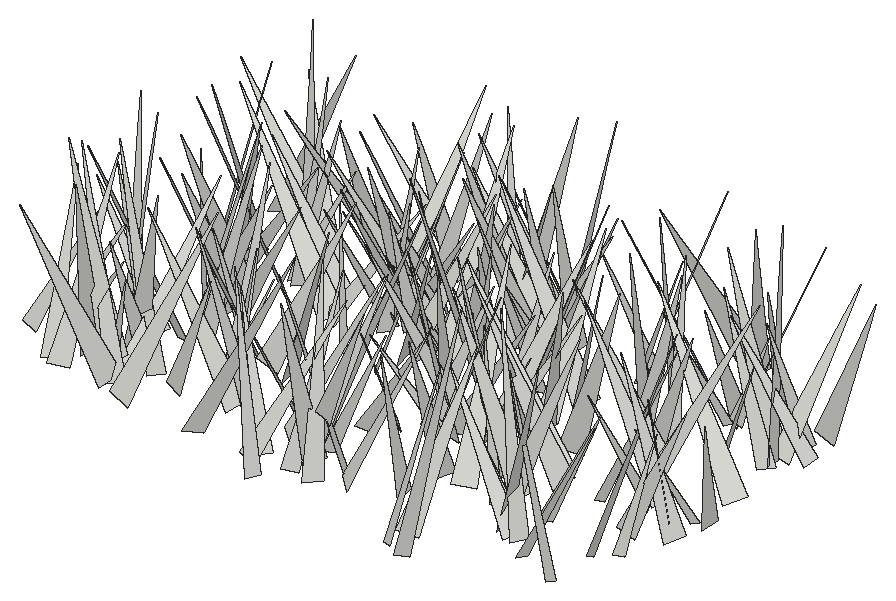
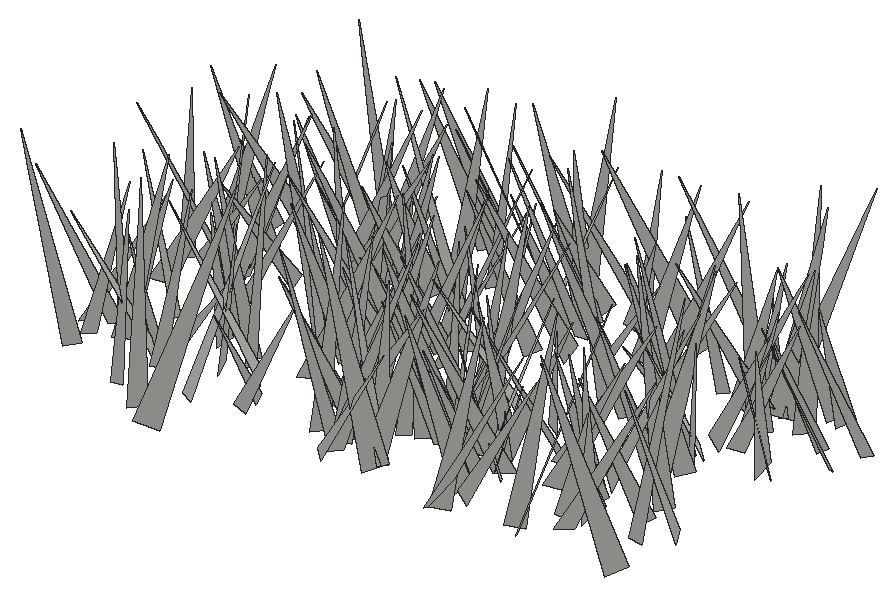
# SketchUp Ruby script. Lengths in inches.
U = 1.inch
M = Sketchup.active_model
def pt(a) = Geom::Point3d.new(a.map { |v| v * U })
def face(e, loops, mat)
  f = e.add_face(loops[0].map { |a| pt(a) })
  loops[1..].each { |l| e.add_face(l.map { |a| pt(a) }).erase! }
  f.material = f.back_material = mat if mat
  f
end
# faces: each face lists its corners as indices into pts; further lists are holes
def faces(e, pts, list, mat = nil) = list.each { |f| face(e, (f[0].is_a?(Array) ? f : [f]).map { |l| l.map { |i| pts[i] } }, mat) }
# xy, xz, yz: faces in a plane at the given z, y or x. An outline is a flat list of corners, or four numbers for a rectangle; further outlines are holes
def ring(l) = l.size == 4 ? [[l[0], l[1]], [l[2], l[1]], [l[2], l[3]], [l[0], l[3]]] : l.each_slice(2).to_a
def flat(e, list, mat, &to3) = list.each { |f| face(e, (f[0].is_a?(Array) ? f : [f]).map { |l| ring(l).map { |u, v| to3.(u, v) } }, mat) }
def xy(e, z, list, mat = nil) = flat(e, list, mat) { |x, y| [x, y, z] }
def xz(e, y, list, mat = nil) = flat(e, list, mat) { |x, z| [x, y, z] }
def yz(e, x, list, mat = nil) = flat(e, list, mat) { |y, z| [x, y, z] }
def lines(e, pts, list) = list.each { |a, b| e.add_line(pt(pts[a]), pt(pts[b])) }
# prism: a flat outline (further loops are holes) pulled along v
def prism(e, loops, v, mat = nil)
  f = face(e, loops, mat); d = Geom::Vector3d.new(v.map { |x| x * U })
  f.pushpull(f.normal.samedirection?(d) ? d.length : -d.length)
end
def box(e, o, s, mat = nil) = prism(e, [[o, [o[0] + s[0], o[1], o[2]], [o[0] + s[0], o[1] + s[1], o[2]], [o[0], o[1] + s[1], o[2]]]], [0, 0, s[2]], mat)
def at(x, y, z, deg = 0) = Geom::Transformation.translation(pt([x, y, z])) * Geom::Transformation.rotation(ORIGIN, Z_AXIS, deg.degrees)
def axes(o, x, y, z) = Geom::Transformation.new([*x, 0, *y, 0, *z, 0, *pt(o).to_a, 1])
def part(name) = M.definitions.add(name)
# library, detail: a bought-in or finely detailed component or shape, given as its bounding box
def library(name, o, s) = part(name).tap { |d| box(d.entities, o, s) }
def detail(e, o, s) = box(e.add_group.entities, o, s)
def put(e, d, t, mat = nil) = e.add_instance(d, t).tap { |i| i.material = mat if mat }
def group(e, t, mat = nil) = e.add_group.tap { |g| g.transformation = t; g.material = mat if mat }.entities
root = M.entities
c1 = part("fur_instance\#9")
p = [[0.8125,0,1.79],[0.67,-0.02,1.48],[0,-0.11,0],[0,0.11,0]]
faces(c1.entities,p,[[0,1,2,3]])
put(root,c1,axes([534.16,231.74,-21.66],[3.4696,4.95294,0.18512],[4.68916,-3.35343,1.83583],[-1.60551,0.90933,5.7619]))
put(root,c1,axes([507.08,237.35,-21.66],[-7.12654,1.94071,2.81889],[3.04033,6.57978,3.15641],[1.57127,-3.9294,6.67765]))
put(root,c1,axes([522.04,233.22,-21.66],[-6.81045,0.95525,0.6863],[0.79996,6.71798,-1.4123],[0.86231,1.31226,6.73054]))
put(root,c1,axes([523.93,237.23,-21.66],[5.76412,-4.56343,1.38579],[-4.26746,-5.90574,-1.69745],[-2.12934,-0.51736,7.15322]))
put(root,c1,axes([535.9,231.1,-21.66],[7.29611,1.84526,3.54482],[-0.04664,-7.33917,3.91643],[-3.99607,3.45479,6.4265]))
put(root,c1,axes([534.38,233.61,-21.66],[-2.83058,6.09964,1.95872],[5.76034,3.3604,-2.14023],[2.80369,-0.74599,6.37473]))
put(root,c1,axes([531.0625,237.41,-21.66],[5.81845,-0.62274,2.18855],[-0.03101,-6.03017,-1.6334],[-2.27522,-1.51035,5.61909]))
put(root,c1,axes([523.18,237.3,-21.66],[5.01421,-5.55154,0.43768],[-5.45899,-4.78379,1.86233],[1.10028,1.565,7.24525]))
put(root,c1,axes([545.39,234.48,-21.66],[-6.80362,-1.51626,0.05987],[-1.39466,6.13985,-2.9915],[-0.59797,2.93174,6.29597]))
put(root,c1,axes([520.3,234.8,-21.66],[1.42855,6.69806,0.59183],[6.31436,-1.12829,-2.47201],[2.31152,-1.05735,6.38701]))
put(root,c1,axes([515.41,235.4,-21.66],[7.23014,-2.66142,0.8801],[-2.79977,-6.73645,2.62947],[0.1379,2.76941,7.24182]))
put(root,c1,axes([538.4,238.49,-21.66],[7.85727,-0.11013,0.63762],[0.0287,-7.70188,-1.68396],[-0.64642,-1.6806,7.67549]))
put(root,c1,axes([527.13,236.25,-21.66],[4.92095,5.18553,0.33695],[5.09859,-4.72846,-1.69263],[1.00379,-1.4039,6.94554]))
put(root,c1,axes([525.42,235.13,-21.66],[-6.65914,2.85732,1.17721],[2.6023,6.69305,-1.52492],[1.66678,0.96593,7.084]))
put(root,c1,axes([541.93,235.84,-21.66],[5.39304,-0.33096,0.39775],[-0.43435,-5.15892,1.59671],[-0.28121,1.6213,5.16187]))
put(root,c1,axes([509.06,235.76,-21.66],[1.74287,7.71217,1.36191],[7.45298,-1.20484,-2.71503],[2.4053,-1.85492,7.42588]))
put(root,c1,axes([503.64,239.86,-21.66],[7.57168,-2.77915,1.4038],[-2.39268,-7.55557,-2.05259],[-1.99233,-1.48808,7.80006]))
put(root,c1,axes([539.83,237.49,-21.66],[-4.53112,4.00144,0.54603],[3.94801,4.21612,1.86503],[-0.85024,-1.74745,5.75015]))
put(root,c1,axes([526.09,237.63,-21.66],[-5.87124,-3.56524,0.53214],[-3.58838,5.68376,-1.51131],[-0.34307,1.5651,6.70063]))
put(root,c1,axes([520.78,236.04,-21.66],[-1.18961,5.30841,0.21099],[4.92708,1.02155,2.07828],[-1.98686,-0.64508,5.02744]))
put(root,c1,axes([510.92,239.01,-21.66],[-0.06945,-5.66946,1.63507],[-5.27402,0.7929,2.5253],[2.64594,1.43164,5.07647]))
put(root,c1,axes([531.5,240.96,-21.66],[5.49992,-4.64771,0.52674],[-4.40214,-5.41809,-1.84207],[-1.58109,-1.08206,6.96111]))
put(root,c1,axes([505.89,239.15,-21.66],[-0.58442,-4.16845,1.10453],[-3.96593,0.95723,1.51414],[1.69333,0.80327,3.92746]))
put(root,c1,axes([517.53,239.08,-21.66],[-1.28539,6.13898,3.44989],[6.89976,0.39684,1.86462],[-1.40785,-3.66012,5.98853]))
put(root,c1,axes([515.48,239.77,-21.66],[-6.93796,2.79801,1.11968],[3.01121,6.55067,2.28891],[0.12298,-2.54512,7.12215]))
put(root,c1,axes([506.13,239.15,-21.66],[-4.3642,6.37446,3.0679],[7.06974,4.05938,1.62241],[0.25406,-3.46117,7.553]))
put(root,c1,axes([523.39,235.33,-21.66],[-6.0414,2.82747,0.77084],[2.14541,5.47009,-3.25002],[1.99649,2.67784,5.82499]))
put(root,c1,axes([540.51,237.37,-21.66],[-7.44461,1.33123,0.56849],[1.18187,7.30967,-1.63995],[0.83578,1.52121,7.38274]))
put(root,c1,axes([506.66,241.51,-21.66],[4.42124,-3.27,0.9733],[-2.9097,-4.44582,-1.71927],[-1.78153,-0.85401,5.22344]))
put(root,c1,axes([523.77,238.8125,-21.66],[4.38543,-2.43855,0.87514],[-2.59033,-4.09309,1.5752],[0.05089,1.80126,4.76417]))
put(root,c1,axes([507.56,237.33,-21.66],[-0.98442,7.82804,0.7856],[7.24103,0.59195,3.17514],[-3.07617,-1.11168,7.22258]))
put(root,c1,axes([520.4375,238.82,-21.66],[4.59981,5.90875,0.46757],[5.722,-4.27232,-2.30133],[1.54616,-1.76752,7.12569]))
put(root,c1,axes([503.27,236.85,-21.66],[-5.30404,4.85737,1.41696],[4.30663,5.41145,-2.42976],[2.65607,0.92563,6.76928]))
put(root,c1,axes([505.93,241.54,-21.66],[3.30529,-7.09092,0.75642],[-7.06387,-3.14139,1.41833],[0.97724,1.27626,7.69379]))
put(root,c1,axes([502.29,237.26,-21.66],[-5.42402,3.35952,0.54018],[3.08821,5.28712,-1.87283],[1.42868,1.32596,6.09909]))
put(root,c1,axes([522.53,238.99,-21.66],[2.40606,6.39383,1.08481],[6.38564,-2.13376,-1.58675],[1.13207,-1.55339,6.64473]))
put(root,c1,axes([498.61,239.65,-21.66],[0.87918,5.14411,1.43079],[4.85097,-0.16366,-2.39235],[2.23095,-1.67133,4.63805]))
put(root,c1,axes([536.82,240.57,-21.66],[-2.52237,2.99386,0.77548],[2.99232,2.10973,1.58806],[-0.78138,-1.58517,3.57821]))
put(root,c1,axes([540.13,240.44,-21.66],[4.26333,-3.02404,0.31767],[-2.97687,-4.03955,1.49732],[0.61963,1.39963,5.00788]))
put(root,c1,axes([519.09,241.4375,-21.66],[-2.36065,-3.34559,0.0438],[-3.13879,2.19578,-1.44709],[-1.15883,0.86782,3.83035]))
put(root,c1,axes([501.26,240.91,-21.66],[2.74116,-2.85153,0.16279],[-2.64199,-2.44575,1.64616],[1.08517,1.2485,3.59657]))
put(root,c1,axes([537.125,241.9375,-21.66],[-7.26006,2.55391,1.83228],[2.95803,7.11093,1.80912],[1.0629,-2.34529,7.48051]))
put(root,c1,axes([529.85,241.97,-21.66],[8.09633,1.85359,0.38508],[1.89305,-7.94545,-1.5559],[-0.02113,-1.6027,8.15877]))
put(root,c1,axes([536.59,241.28,-21.66],[1.17731,-6.81979,2.88625],[-6.91612,0.0321,2.89694],[2.64712,3.11697,6.28517]))
put(root,c1,axes([546.7,239.78,-21.66],[3.7026,-0.58317,1.91769],[-1.4169,-3.61072,1.63767],[-1.41775,2.08554,3.37155]))
put(root,c1,axes([508.91,239.76,-21.66],[-0.71343,7.62578,1.29035],[7.14993,0.15622,3.02994],[-2.94889,-1.46615,7.03427]))
put(root,c1,axes([545.24,242.32,-21.66],[1.83372,-5.8574,1.52699],[-5.60076,-1.03656,2.74963],[2.29617,2.14936,5.48737]))
put(root,c1,axes([525.13,244.25,-21.66],[-2.98193,-4.15353,0.46379],[-3.81224,2.9367,1.78925],[1.71281,-0.69483,4.78981]))
put(root,c1,axes([523.67,242.54,-21.66],[3.57334,-4.4658,0.19156],[-4.12422,-3.19939,2.34597],[1.72363,1.60293,5.21618]))
put(root,c1,axes([507.09,239.3,-21.66],[-0.93463,7.10607,0.24964],[6.82555,0.96718,-1.97702],[1.99262,0.02006,6.88921]))
put(root,c1,axes([536.3125,240.22,-21.66],[-5.7713,0.32455,0.04644],[0.28097,5.31808,-2.2482],[0.16895,2.24233,5.3253]))
put(root,c1,axes([545.32,238.625,-21.66],[6.83312,3.40706,1.30672],[2.45514,-6.34476,3.70451],[-2.69961,2.8536,6.67654]))
put(root,c1,axes([528.7,244.81,-21.66],[-4.92347,-1.39259,0.14711],[-1.23579,4.5738,1.93769],[0.65861,-1.82825,4.73553]))
put(root,c1,axes([507.3,241.24,-21.66],[-6.47288,0.26814,0.01301],[0.25719,6.28405,-1.55397],[0.07694,1.55212,6.2893]))
put(root,c1,axes([548.21,243.64,-21.66],[-6.07802,2.92755,1.98205],[3.37511,5.97833,1.51972],[1.05246,-2.26504,6.57292]))
put(root,c1,axes([513.8,241.26,-21.66],[4.21835,1.12148,1.8478],[0.48542,-4.44001,1.58659],[-2.10629,1.22277,4.06632]))
put(root,c1,axes([499.32,242.52,-21.66],[3.29682,4.04593,0.27696],[3.82738,-2.98619,-1.93627],[1.34069,-1.42422,4.84659]))
put(root,c1,axes([507.35,244.4,-21.66],[-3.5976,-6.50533,0.64098],[-6.34012,3.29439,-2.15004],[-1.59153,1.58132,7.11613]))
put(root,c1,axes([534.4,243.14,-21.66],[0.81184,5.62301,2.88886],[5.96448,-1.64652,1.52868],[-2.09495,-2.50871,5.47179]))
put(root,c1,axes([515.63,245,-21.66],[7.87771,-0.03675,0.30438],[0.03502,-7.66773,-1.83222],[-0.30459,-1.83219,7.66177]))
put(root,c1,axes([538.15,244.85,-21.66],[-7.32197,2.2534,1.35544],[2.57225,6.97064,2.30649],[0.54639,-2.61889,7.30542]))
put(root,c1,axes([544.14,246.11,-21.66],[-5.03232,-2.4099,0.87584],[-1.92345,4.82363,2.22078],[1.6956,-1.68045,5.11859]))
put(root,c1,axes([546.28,245.39,-21.66],[-3.5454,-4.09399,1.47684],[-3.82101,3.83994,1.47185],[2.08366,0.07566,5.21193]))
put(root,c1,axes([521.68,241.16,-21.66],[7.63616,1.08232,1.22596],[0.61242,-7.3209,2.64853],[-1.51635,2.49367,7.24345]))
put(root,c1,axes([505.67,244.31,-21.66],[-4.20776,3.77593,1.0344],[3.85861,3.7428,2.0336],[-0.66241,-2.18328,5.27517]))
put(root,c1,axes([512.74,242.02,-21.66],[-3.04551,1.64304,1.0176],[0.80196,2.80235,-2.12461],[1.7584,1.56764,2.73144]))
put(root,c1,axes([513.96,240.83,-21.66],[-7.01528,2.7432,0.95764],[2.14491,6.5776,-3.12905],[1.96,2.6204,6.85188]))
put(root,c1,axes([533.31,240.64,-21.66],[-6.01479,5.28528,0.0687],[5.03484,5.76049,-2.36301],[1.60915,1.73181,7.65037]))
put(root,c1,axes([533.56,247.27,-21.66],[5.51839,-2.97407,0.09463],[-2.75984,-5.19025,-2.17974],[-1.11235,-1.87694,5.87762]))
put(root,c1,axes([533.8125,243.97,-21.66],[0.77097,6.55392,2.92574],[6.60675,-1.79779,2.28627],[-2.8044,-2.43357,6.19042]))
put(root,c1,axes([548.8,246.48,-21.66],[5.13341,-1.95182,0.40555],[-1.78394,-4.9977,-1.47188],[-0.88973,-1.24068,5.29103]))
put(root,c1,axes([529.16,245,-21.66],[-3.64938,-5.29226,1.74557],[-5.55344,3.28039,-1.66476],[-0.463,2.36729,6.20923]))
put(root,c1,axes([527.09,244.8,-21.66],[1.94999,6.06367,1.85826],[6.06829,-1.21894,-2.39034],[1.84311,-2.40204,5.90397]))
put(root,c1,axes([512.32,245.74,-21.66],[-4.6508,-5.63712,0.37429],[-5.36466,4.25457,-2.58191],[-1.77136,1.91537,6.83673]))
put(root,c1,axes([527.18,247.84,-21.66],[-7.29024,-1.74958,0.87658],[-1.40156,7.02793,2.37084],[1.36568,-2.12702,7.11251]))
put(root,c1,axes([547.84,246.15,-21.66],[-0.53868,-3.7535,0.51973],[-3.36849,0.23389,-1.80211],[-1.73555,0.71104,3.33637]))
put(root,c1,axes([511.94,245.49,-21.66],[-1.05055,-3.99645,1.56356],[-4.12582,0.49771,-1.49997],[-1.18067,1.81677,3.85037]))
put(root,c1,axes([537.49,245.73,-21.66],[-6.42815,4.45601,0.04956],[4.21627,6.0534,2.59983],[-1.44275,-2.16333,7.37686]))
put(root,c1,axes([513.7,245.12,-21.66],[0.25719,7.17904,2.90731],[6.91163,1.10018,-3.3281],[3.49578,-2.70337,6.36621]))
put(root,c1,axes([528.39,245.79,-21.66],[4.87522,-3.55324,0.35007],[-3.38958,-4.41978,2.34354],[1.12198,2.08707,5.55888]))
put(root,c1,axes([544.53,247,-21.66],[-6.88709,2.46248,0.81316],[2.58785,6.67518,1.70354],[0.16756,-1.88022,7.11293]))
put(root,c1,axes([531.35,244.49,-21.66],[3.64416,1.65962,0.06909],[1.4569,-3.27351,1.789],[-0.79783,1.60274,3.58241]))
put(root,c1,axes([507.73,246.48,-21.66],[2.9133,6.77269,2.26525],[7.08174,-2.424,-1.8604],[0.9217,-2.7826,7.13411]))
put(root,c1,axes([507.59,249.75,-21.66],[5.40513,-4.44008,1.03103],[-3.91993,-5.34397,-2.46351],[-2.32626,-1.31164,6.54682]))
put(root,c1,axes([531.17,246.39,-21.66],[2.97178,5.39968,0.42783],[5.06638,-2.59832,-2.39825],[1.91609,-1.5044,5.67771]))
put(root,c1,axes([535.83,248.48,-21.66],[4.04324,-6.81137,0.9787],[-6.74817,-3.70246,2.11055],[1.34718,1.89668,7.63467]))
put(root,c1,axes([541.24,244.67,-21.66],[5.35308,0.77922,1.1136],[0.09871,-4.73607,2.83947],[-1.35556,2.73224,4.60435]))
put(root,c1,axes([533.02,249.5625,-21.66],[7.23074,-0.77372,0.74856],[-0.57311,-7.06946,-1.77111],[-0.91134,-1.69312,7.05304]))
put(root,c1,axes([506.23,248.78,-21.66],[2.55754,-6.5759,0.86107],[-6.14173,-2.00015,2.96707],[2.50263,1.81158,6.40156]))
put(root,c1,axes([502.31,245.2,-21.66],[3.51213,5.3509,1.08193],[4.75447,-3.63032,2.52063],[-2.68285,0.57134,5.88334]))
put(root,c1,axes([502.63,245.3,-21.66],[-7.06937,0.92542,0.80535],[0.55425,6.6114,-2.73188],[1.09444,2.62944,6.58553]))
put(root,c1,axes([506.96,247.23,-21.66],[2.66286,4.62658,1.9724],[4.32664,-3.24515,1.77077],[-2.56433,-0.67099,5.03592]))
put(root,c1,axes([530.92,246.67,-21.66],[-0.22471,7.89617,1.63504],[7.5306,0.79034,-2.78188],[2.88322,-1.44886,7.39332]))
put(root,c1,axes([506.36,251.9375,-21.66],[4.04445,-6.42376,0.8146],[-6.13253,-4.10829,-1.94934],[-2.07854,-0.37835,7.33638]))
put(root,c1,axes([507.27,245.83,-21.66],[4.44404,5.53922,0.27989],[5.13876,-4.2472,2.46279],[-2.08674,1.3376,6.66087]))
put(root,c1,axes([520.01,251.13,-21.66],[6.41369,-0.07562,0.05633],[-0.05586,-6.13403,-1.87481],[-0.07597,-1.87412,6.13403]))
put(root,c1,axes([523.32,251.26,-21.66],[5.23051,-1.10724,0.78196],[-0.81536,-5.06,-1.7109],[-1.08287,-1.53819,5.06527]))
put(root,c1,axes([528.1,249.67,-21.66],[-4.4516,-6.59475,1.62319],[-6.65602,3.85048,-2.61027],[-1.35017,2.76139,7.51625]))
put(root,c1,axes([507.82,249.86,-21.66],[4.10331,-3.61689,0.17449],[-3.47529,-3.85943,1.7253],[1.0172,1.40442,5.19061]))
put(root,c1,axes([533.65,251.42,-21.66],[7.53646,1.85279,1.2332],[2.16443,-7.11553,-2.53698],[-0.51849,-2.77277,7.33449]))
put(root,c1,axes([541.34,251,-21.66],[-6.98354,0.71492,0.27676],[0.75932,6.7998,1.59491],[0.10557,-1.6153,6.83646]))
put(root,c1,axes([520.72,252.91,-21.66],[0.06912,-7.57158,0.2529],[-7.42195,-0.11839,-1.51598],[-1.51902,0.23392,7.41859]))
put(root,c1,axes([520.83,251.98,-21.66],[5.55902,-2.83125,1.90418],[-2.404,-5.83322,-1.65498],[-2.42129,-0.70867,6.01496]))
put(root,c1,axes([542.3,248.66,-21.66],[3.82071,6.83533,0.31448],[6.59967,-3.58608,-2.23672],[1.80694,-1.35528,7.50444]))
put(root,c1,axes([548.06,249.99,-21.66],[-5.28258,5.45364,0.12335],[5.18528,4.96674,2.47132],[-1.69419,-1.80343,7.17917]))
put(root,c1,axes([516.51,249.42,-21.66],[1.26657,4.59176,1.22685],[4.36989,-1.62436,1.56816],[-1.86909,-0.68616,4.4977]))
put(root,c1,axes([539.9,251.875,-21.66],[2.36521,-5.47601,0.71506],[-5.30162,-2.03369,1.96193],[1.54624,1.40343,5.6331]))
put(root,c1,axes([524.92,252.29,-21.66],[-1.49518,-5.85947,1.8909],[-5.5495,2.12534,2.19783],[2.66683,1.13753,5.63369]))
put(root,c1,axes([504.42,253.1875,-21.66],[8.18505,-1.50624,0.16494],[-1.43272,-7.98824,-1.85106],[-0.49323,-1.79175,8.11402]))
put(root,c1,axes([531.82,247.43,-21.66],[7.42778,3.7642,0.92799],[3.25227,-7.14156,2.93652],[-2.11023,2.24305,7.79217]))
put(root,c1,axes([521.25,253.78,-21.66],[-3.70308,-3.24105,0.05421],[-3.08159,3.54543,1.46762],[1.00557,-1.07036,4.69716]))
put(root,c1,axes([518.14,254.93,-21.66],[6.29678,-5.28708,1.00032],[-4.88133,-6.26054,-2.36253],[-2.26416,-1.20654,7.87535]))
put(root,c1,axes([509.29,252.6875,-21.66],[-4.9129,-5.75828,0.52895],[-5.68371,4.68095,-1.83254],[-1.06438,1.58274,7.34412]))
put(root,c1,axes([544.375,253.02,-21.66],[5.4983,0.81734,0.21266],[0.84397,-5.26527,-1.58403],[0.03145,-1.59793,5.32824]))
put(root,c1,axes([520.83,254.45,-21.66],[-8.10416,-1.22815,0.06312],[-1.16757,7.81624,2.17553],[0.38615,-2.14192,7.90272]))
put(root,c1,axes([516.7,254.12,-21.66],[0.11807,-5.18176,0.38422],[-4.95689,-0.22756,-1.54584],[-1.55804,0.33133,4.94722]))
put(root,c1,axes([529.51,253.34,-21.66],[-1.62801,-6.13851,1.48062],[-6.15059,1.19536,-1.80699],[-1.42958,1.84764,6.08822]))
put(root,c1,axes([517.17,255.42,-21.66],[-4.17954,-4.03403,0.06779],[-3.83281,4.00041,1.74723],[1.26,-1.21235,5.53978]))
put(root,c1,axes([532,250.76,-21.66],[-2.25135,6.36064,1.32657],[6.19225,2.52565,-1.60099],[1.96812,-0.67041,6.55463]))
put(root,c1,axes([519.65,248.7,-21.66],[5.70548,5.18554,0.14342],[4.71826,-5.27598,3.06024],[-2.15603,2.1765,7.07653]))
put(root,c1,axes([528.83,251.14,-21.66],[-4.17558,2.72173,1.55923],[2.19552,4.39009,-1.78362],[2.24025,0.77057,4.65424]))
put(root,c1,axes([522.16,255.45,-21.66],[0.1957,-7.90399,1.09327],[-7.43409,0.21668,2.89722],[2.89871,1.0893,7.35646]))
put(root,c1,axes([512.96,252.6,-21.66],[-5.23637,6.32875,0.17784],[5.87309,4.76933,3.20385],[-2.36465,-2.16904,7.5636]))
put(root,c1,axes([513.02,252.4,-21.66],[2.725,5.40327,0.30402],[4.86473,-2.29653,-2.78814],[2.3711,-1.498,5.37096]))
put(root,c1,axes([532.75,253.96,-21.66],[-7.09229,4.18803,1.11711],[4.32642,6.70959,2.31334],[-0.26383,-2.55536,7.90497]))
put(root,c1,axes([536.72,255.01,-21.66],[6.67439,0.3641,2.55328],[0.99441,-6.8993,-1.61558],[-2.3797,-1.86182,6.48614]))
put(root,c1,axes([537.26,254.09,-21.66],[0.1838,-6.38239,2.38865],[-6.46729,0.58989,2.0738],[2.14821,2.32195,6.03888]))
put(root,c1,axes([516.36,254.3,-21.66],[-1.2496,-4.95098,2.04852],[-4.91628,1.89585,1.58307],[2.13046,1.47094,4.85465]))
put(root,c1,axes([519.625,252.66,-21.66],[0.86928,6.52033,1.58307],[6.24969,-0.2059,-2.58369],[2.44176,-1.79425,6.04937]))
put(root,c1,axes([529.21,255.7,-21.66],[1.40326,-4.201,0.43994],[-3.89786,-1.46649,-1.57071],[-1.62745,-0.10993,4.1413]))
put(root,c1,axes([523.49,255.92,-21.66],[4.86782,-2.47433,0.4659],[-2.27673,-4.75873,-1.48527],[-1.07512,-1.1257,5.25471]))
put(root,c1,axes([503.3,257.53,-21.66],[-3.16063,-7.46069,0.64697],[-7.21635,3.22195,1.90087],[2.00118,-0.16476,7.87643]))
put(root,c1,axes([518.74,257.26,-21.66],[-3.46675,-5.54657,1.13696],[-5.08588,3.63649,2.23277],[2.48816,-0.29493,6.14797]))
put(root,c1,axes([511.83,255.3,-21.66],[-4.61226,3.61546,0.79034],[3.61757,4.1381,2.18138],[-0.78062,-2.18488,5.43931]))
put(root,c1,axes([516.79,253.24,-21.66],[-5.68198,1.58826,2.45655],[1.00817,6.10119,-1.61279],[2.74605,1.04639,5.67506]))
put(root,c1,axes([525.66,257.53,-21.66],[3.52912,-6.81057,1.30534],[-6.45742,-3.76145,-2.16695],[-2.52774,0.10047,7.35818]))
put(root,c1,axes([546.97,254.52,-21.66],[-2.40654,5.51072,1.54274],[5.60544,1.9331,1.83892],[-1.15197,-2.10585,5.72519]))
put(root,c1,axes([517.65,257.98,-21.66],[-5.63617,-2.55407,1.20627],[-1.85262,5.37498,2.72438],[2.13217,-2.08115,5.55585]))
put(root,c1,axes([520.44,254.01,-21.66],[6.21247,-1.9108,0.54363],[-1.98453,-5.88708,1.9863],[0.09123,2.05733,6.18874]))
put(root,c1,axes([504.27,255.07,-21.66],[3.95823,-3.37287,0.12226],[-3.1364,-3.60629,2.0534],[1.24667,1.63622,4.7778]))
put(root,c1,axes([539.9,253.7,-21.66],[-5.67085,1.89535,1.35099],[1.57668,5.74544,-1.44226],[1.71219,0.98676,5.80265]))
put(root,c1,axes([507.76,255.28,-21.66],[2.74788,4.31889,0.7575],[4.17328,-2.30167,-2.01583],[1.34551,-1.68135,4.70533]))
put(root,c1,axes([522.2,253.07,-21.66],[-3.86216,7.0455,1.20437],[6.7899,4.04407,-1.88376],[2.2331,-0.11104,7.81068]))
put(root,c1,axes([548.68,256.89,-21.66],[-5.67147,0.82087,0.04901],[0.80443,5.46726,1.5178],[-0.17066,-1.50898,5.5259]))
put(root,c1,axes([508.2,254.95,-21.66],[5.34451,-1.51745,2.02584],[-2.07356,-5.33917,1.4711],[-1.45157,2.03988,5.35746]))
put(root,c1,axes([520.91,255.42,-21.66],[0.51844,5.23573,1.343],[5.13497,-0.0558,-1.76472],[1.68777,-1.43851,4.95655]))
put(root,c1,axes([516.24,255.46,-21.66],[-4.21104,-1.2398,0.43934],[-1.31531,3.95873,-1.43574],[-0.00925,1.50143,4.14832]))
put(root,c1,axes([541.25,258.89,-21.66],[5.27025,-2.47106,0.85487],[-2.00329,-5.05203,-2.25305],[-1.68041,-1.72721,5.36707]))
put(root,c1,axes([514.88,256.73,-21.66],[3.85978,2.30102,0.3483],[2.28006,-3.60384,-1.45862],[0.46617,-1.42533,4.2503]))
put(root,c1,axes([547.47,258.12,-21.66],[-4.78026,1.17069,2.19317],[1.89155,4.79719,1.56216],[1.61324,-2.15588,4.66702]))
put(root,c1,axes([545.3,257.29,-21.66],[3.76435,-5.16952,3.38659],[-5.24976,-4.76711,-1.44149],[-3.26082,1.70703,6.23028]))
put(root,c1,axes([508.73,254.49,-21.66],[-6.51752,1.2418,2.00991],[0.54856,6.53189,-2.25684],[2.29801,1.9627,6.23913]))
put(root,c1,axes([509.04,257.15,-21.66],[-3.24563,2.42896,0.17461],[2.25293,2.88449,1.75171],[-0.92447,-1.49811,3.65588]))
put(root,c1,axes([527.98,258.9,-21.66],[6.98441,-2.34407,2.00985],[-1.86712,-7.16517,-1.86827],[-2.45928,-1.21733,7.12645]))
put(root,c1,axes([541.52,257.46,-21.66],[-1.12844,-4.06047,0.83548],[-3.60524,0.5338,-2.27512],[-2.04639,1.29864,3.54749]))
put(root,c1,axes([546.91,255.29,-21.66],[-7.37531,-1.40171,2.74866],[-2.16749,7.42249,-2.03071],[2.19589,2.61858,7.22747]))
put(root,c1,axes([516.49,257.01,-21.66],[3.7348,-2.45498,0.02516],[-2.33086,-3.53122,1.44009],[0.77113,1.21649,4.23106]))
put(root,c1,axes([537.35,260.74,-21.66],[-4.65731,-6.85842,0.0184],[-6.74044,4.58127,1.51895],[1.26677,-0.83835,8.14992]))
put(root,c1,axes([525.89,259.28,-21.66],[5.91516,-3.3432,1.65321],[-2.9566,-6.09276,-1.74243],[-2.27346,-0.77492,6.56735]))
put(root,c1,axes([509.72,261.66,-21.66],[-6.50454,-4.83681,0.42708],[-4.2184,5.98256,3.50717],[2.40464,-2.5885,7.30777]))
put(root,c1,axes([501.47,255.45,-21.66],[5.51365,3.20537,1.24598],[2.89904,-5.59864,1.57419],[-1.84998,0.77981,6.18035]))
put(root,c1,axes([537.99,256.39,-21.66],[-6.10428,-1.79449,1.71008],[-2.20054,6.01533,-1.54278],[1.14113,2.0006,6.1727]))
put(root,c1,axes([541.73,257.95,-21.66],[0.78956,-4.05986,1.16414],[-3.93825,-0.27989,1.69498],[1.52574,1.37851,3.77266]))
put(root,c1,axes([527.8,255.95,-21.66],[5.78446,0.51407,0.77192],[0.25637,-5.57234,1.78981],[-0.89129,1.73346,5.52457]))
put(root,c1,axes([523.09,259.55,-21.66],[1.43067,-7.01564,1.7352],[-6.90944,-1.84641,-1.76845],[-2.11892,1.28394,6.9382]))
put(root,c1,axes([527.23,257.87,-21.66],[-4.14935,5.21761,0.66717],[4.85978,3.47746,3.02911],[-2.01273,-2.35998,5.93844]))
put(root,c1,axes([510.45,260.88,-21.66],[5.40488,-4.57462,0.50738],[-4.27322,-5.27816,-2.06831],[-1.71004,-1.26929,6.77215]))
put(root,c1,axes([522.02,259.92,-21.66],[7.41722,0.99885,0.34739],[1.05742,-6.96886,-2.53978],[0.01548,-2.56338,7.04006]))
put(root,c1,axes([546.83,256.06,-21.66],[0.07577,6.70614,0.84141],[6.48392,0.16538,-1.90197],[1.90764,-0.82847,6.43122]))
put(root,c1,axes([525.54,257.91,-21.66],[4.06898,-3.86093,0.67624],[-3.71406,-3.48612,2.44405],[1.25293,2.20473,5.04877]))
put(root,c1,axes([525.66,260.37,-21.66],[-7.8024,0.71377,1.7229],[1.19599,7.6017,2.26696],[1.43089,-2.46171,7.49986]))
put(root,c1,axes([507.84,259.0625,-21.66],[-6.653,2.83628,0.09553],[2.75112,6.38619,1.99099],[-0.69638,-1.86767,6.95291]))
put(root,c1,axes([535.25,255.84,-21.66],[6.47525,4.61232,0.40047],[4.47579,-6.41261,1.48613],[-1.18373,0.98374,7.80985]))
put(root,c1,axes([515.37,255.76,-21.66],[-1.37451,8.097,0.63904],[7.82187,1.49419,-2.10823],[2.18815,-0.25501,7.93763]))
put(root,c1,axes([547.38,259.93,-21.66],[1.03631,-6.95808,1.71035],[-6.57848,-0.23906,3.0134],[2.83968,1.98547,6.35675]))
put(root,c1,axes([524.68,256.9,-21.66],[-0.02832,7.80203,1.3013],[7.5934,-0.33756,2.1891],[-2.2148,-1.25708,7.48868]))
put(root,c1,axes([507.48,256.87,-21.66],[-7.86516,0.65945,1.92725],[0.13584,7.83978,-2.12819],[2.03241,2.02799,7.60042]))
put(root,c1,axes([533.8125,259.81,-21.66],[-0.35504,-4.51922,1.36303],[-4.31721,-0.2418,-1.92625],[-1.90863,1.3876,4.10353]))
put(root,c1,axes([515.41,260.08,-21.66],[-2.41735,-5.08882,0.8159],[-4.81582,1.90935,-2.35956],[-1.83565,1.69223,5.11586]))
put(root,c1,axes([508.69,258.01,-21.66],[-2.09774,5.99421,0.07606],[5.73274,1.98235,1.88224],[-1.75272,-0.69034,6.06533]))
put(root,c1,axes([533.58,258.13,-21.66],[3.9731,1.20771,1.01378],[0.70264,-3.81635,1.79266],[-1.41159,1.49959,3.74573]))
put(root,c1,axes([515.65,262.03,-21.66],[3.87648,-5.20572,1.47803],[-5.00062,-4.14086,-1.46909],[-2.0683,0.2548,6.32205]))
put(root,c1,axes([541.99,262.125,-21.66],[-0.85203,-5.57664,0.61964],[-5.3803,0.98986,1.51043],[1.59225,0.36067,5.43539]))
put(root,c1,axes([542.01,257.83,-21.66],[5.76242,3.50846,0.12226],[3.39302,-5.62636,1.53663],[-0.90093,1.2508,6.56914]))
put(root,c1,axes([516.08,259.16,-21.66],[6.10707,-2.19869,2.10682],[-2.76305,-5.98564,1.76265],[-1.28003,2.43046,6.24689]))
put(root,c1,axes([522.17,260.4375,-21.66],[6.94828,-4.27135,1.74082],[-4.55894,-6.83788,1.41876],[-0.70067,2.13364,8.03182]))
put(root,c1,axes([516.23,262.18,-21.66],[-6.42762,0.7775,0.36666],[0.8533,6.10569,2.01137],[0.10407,-2.04186,6.15412]))
put(root,c1,axes([526.8125,258.97,-21.66],[7.21368,2.51232,2.17903],[2.05011,-7.45745,1.81123],[-2.61859,1.08246,7.42081]))
put(root,c1,axes([526.13,261.27,-21.66],[-3.48224,-3.77241,0.29956],[-3.58403,3.15695,-1.90663],[-1.21472,1.49981,4.76674]))
put(root,c1,axes([537.04,265.27,-21.66],[4.97759,-6.71856,0.2944],[-6.18791,-4.7191,-3.07278],[-2.63353,-1.61035,7.77647]))
put(root,c1,axes([501.76,261.34,-21.66],[6.68383,-3.60485,0.36068],[-3.59385,-6.50181,1.61538],[0.45749,1.59067,7.42019]))
put(root,c1,axes([539.02,263.74,-21.66],[7.15666,-2.1147,0.99823],[-1.83229,-7.06792,-1.83669],[-1.45298,-1.50292,7.233]))
